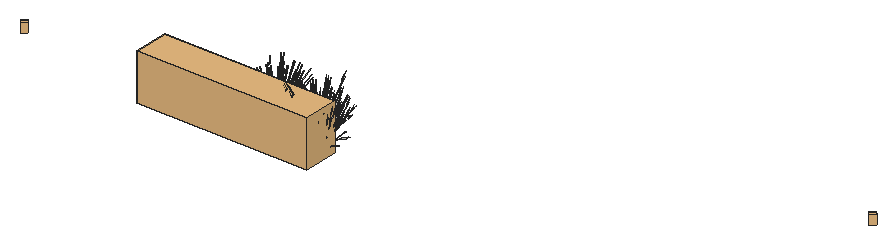
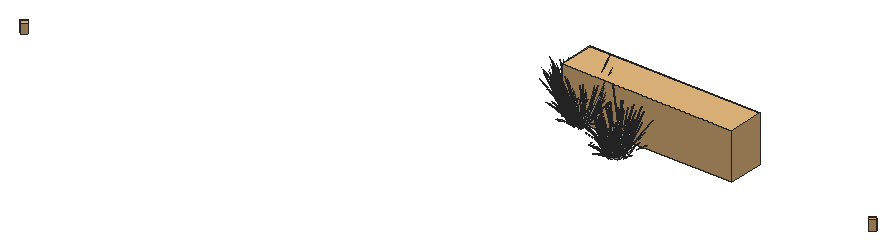
# SketchUp Ruby script. Lengths in inches.
U = 1.inch
M = Sketchup.active_model
def pt(a) = Geom::Point3d.new(a.map { |v| v * U })
def face(e, loops, mat)
  f = e.add_face(loops[0].map { |a| pt(a) })
  loops[1..].each { |l| e.add_face(l.map { |a| pt(a) }).erase! }
  f.material = f.back_material = mat if mat
  f
end
# faces: each face lists its corners as indices into pts; further lists are holes
def faces(e, pts, list, mat = nil) = list.each { |f| face(e, (f[0].is_a?(Array) ? f : [f]).map { |l| l.map { |i| pts[i] } }, mat) }
# xy, xz, yz: faces in a plane at the given z, y or x. An outline is a flat list of corners, or four numbers for a rectangle; further outlines are holes
def ring(l) = l.size == 4 ? [[l[0], l[1]], [l[2], l[1]], [l[2], l[3]], [l[0], l[3]]] : l.each_slice(2).to_a
def flat(e, list, mat, &to3) = list.each { |f| face(e, (f[0].is_a?(Array) ? f : [f]).map { |l| ring(l).map { |u, v| to3.(u, v) } }, mat) }
def xy(e, z, list, mat = nil) = flat(e, list, mat) { |x, y| [x, y, z] }
def xz(e, y, list, mat = nil) = flat(e, list, mat) { |x, z| [x, y, z] }
def yz(e, x, list, mat = nil) = flat(e, list, mat) { |y, z| [x, y, z] }
def lines(e, pts, list) = list.each { |a, b| e.add_line(pt(pts[a]), pt(pts[b])) }
# prism: a flat outline (further loops are holes) pulled along v
def prism(e, loops, v, mat = nil)
  f = face(e, loops, mat); d = Geom::Vector3d.new(v.map { |x| x * U })
  f.pushpull(f.normal.samedirection?(d) ? d.length : -d.length)
end
def box(e, o, s, mat = nil) = prism(e, [[o, [o[0] + s[0], o[1], o[2]], [o[0] + s[0], o[1] + s[1], o[2]], [o[0], o[1] + s[1], o[2]]]], [0, 0, s[2]], mat)
def at(x, y, z, deg = 0) = Geom::Transformation.translation(pt([x, y, z])) * Geom::Transformation.rotation(ORIGIN, Z_AXIS, deg.degrees)
def axes(o, x, y, z) = Geom::Transformation.new([*x, 0, *y, 0, *z, 0, *pt(o).to_a, 1])
def part(name) = M.definitions.add(name)
# library, detail: a bought-in or finely detailed component or shape, given as its bounding box
def library(name, o, s) = part(name).tap { |d| box(d.entities, o, s) }
def detail(e, o, s) = box(e.add_group.entities, o, s)
def put(e, d, t, mat = nil) = e.add_instance(d, t).tap { |i| i.material = mat if mat }
def group(e, t, mat = nil) = e.add_group.tap { |g| g.transformation = t; g.material = mat if mat }.entities
root = M.entities
M.materials.add("LightPink_Translucent").color = [144, 107, 117]
M.materials["LightPink_Translucent"].alpha = 0.75
c1 = part("blade")
p = [[2.15,0.21,22],[0,0.17,0],[0.09,0.45,0],[2.18,0.31,22],[2.29,0.31,22],[0.38,0.45,0],
  [2.48,0.24,33],[2.49,0.24,33],[2.48,0.22,33]]
faces(c1.entities,p,[[0,1,2,3],[4,5,2,3],[6,3,4,7],[8,0,3,6]])
c2 = part("blade with seeds\#1")
put(c2.entities,c1,at(0,0,0))
c3 = part("seeds")
p = [[0.3,-0.1,1.38],[-0.01,-0.03,1.59],[-0.01,-0.03,0.03],[0.14,-0.07,-0.07],[0.29,-0.03,3],[0.15,0.01,3.11]]
faces(c3.entities,p,[[0,1,2,3],[1,0,4,5]],"LightPink_Translucent")
c4 = part("blade with seeds")
put(c4.entities,c1,at(0,0,0))
put(c4.entities,c3,axes([2.4,0.25,30.99],[1.5799,-0.05474,1.17369],[-0.12525,1.92788,0.29478],[-0.07173,-0.02425,1.56792]))
c5 = library("Areca palm plant",[21.56,16.8,2.55],[5.71,6.07,10.56])
c6 = library("Group\#130",[-6.15,-1.2,0],[37.48,180.08,49.04])
c7 = part("PLANTS (1)")
put(c7.entities,c5,axes([-554.71,-75.81,3.93],[0.45017,-0.56191,0],[0.66137,0.52986,0],[0,0,0.72]))
put(c7.entities,c5,axes([38.49,68.02,6.02],[0.45017,-0.56191,0],[0.66137,0.52986,0],[0,0,0.72]))
put(c7.entities,c6,axes([-275.95,-98.77,3.0625],[0,0.79,0],[-0.79,0,0],[0,0,0.79]))
put(root,c2,axes([522.07,92.45,2.78],[-0.61172,0.65782,-0.31925],[-0.57907,-0.75112,0.41216],[-0.08811,0.38163,0.78863]))
put(root,c2,axes([527.67,81.52,2.24],[-0.82131,0.22128,-0.03148],[-0.18882,-1.04586,-0.14272],[0.05207,-0.2184,0.47074]))
put(root,c4,axes([568.41,68.2,4.17],[-1.04497,-0.50058,-0.71045],[0.74264,-0.8772,0.08574],[-0.3786,-0.29889,1.00501]))
put(root,c4,axes([569.55,75.89,4.17],[0.5849,0.8421,-0.71045],[-1.20401,0.4693,0.08574],[0.13677,0.40688,1.00501]))
put(root,c4,axes([566.28,69.43,4.17],[-1.22504,-0.02494,-0.71045],[0.08228,-1.05005,0.08574],[-0.51899,-0.11081,1.00501]))
put(root,c4,axes([575.07,70.45,4.17],[0.64013,-0.81717,-0.71045],[1.12174,0.58074,0.08574],[0.38221,-0.29607,1.00501]))
put(root,c4,axes([575.37,72.51,4.17],[1.07686,-0.45739,-0.71045],[0.60013,0.94154,0.08574],[0.52031,-0.10696,1.00501]))
put(root,c4,axes([573.48,68.78,4.17],[0.03189,-0.95798,-0.71045],[1.34277,0.06434,0.08574],[0.14171,-0.40585,1.00501]))
put(root,c4,axes([574.32,74.41,4.17],[1.22504,0.02494,-0.71045],[-0.08228,1.05005,0.08574],[0.51899,0.11081,1.00501]))
put(root,c4,axes([571.05,67.96,4.17],[-0.5849,-0.8421,-0.71045],[1.20401,-0.4693,0.08574],[-0.13677,-0.40688,1.00501]))
put(root,c2,axes([526.01,85.84,2.19],[-0.16834,0.42944,1.54493],[-0.70619,-0.88871,0.12492],[0.31858,-0.5539,0.66044]))
put(root,c2,axes([521.4,86.39,2.19],[0.33582,0.21526,1.54493],[-0.69497,0.90306,0.12492],[-0.43315,-0.40739,0.66044]))
put(root,c2,axes([524.47,84.9375,2.19],[0.02213,0.47954,1.54493],[-0.95907,-0.31812,0.12492],[0.05932,-0.68338,0.66044]))
put(root,c2,axes([526.99,87.61,2.19],[-0.31369,0.26428,1.54493],[-0.26409,-1.22118,0.12492],[0.49247,-0.276,0.66044]))
put(root,c2,axes([527.15,89.77,2.19],[-0.375,0.0283,1.54493],[0.24877,-1.22643,0.12492],[0.53441,0.07586,0.66044]))
put(root,c2,axes([526.4375,91.74,2.19],[-0.33582,-0.21526,1.54493],[0.69497,-0.90306,0.12492],[0.43315,0.40739,0.66044]))
put(root,c2,axes([525.05,92.99,2.19],[-0.20666,-0.40114,1.54493],[0.95496,-0.33772,0.12492],[0.21583,0.62976,0.66044]))
put(root,c2,axes([525.7,91.52,2.19],[-0.3002,-0.28876,1.54493],[0.81031,-0.72911,0.12492],[0.36902,0.50009,0.66044]))
put(root,c2,axes([520.85,90.51,2.19],[0.31369,-0.26428,1.54493],[0.26409,1.22118,0.12492],[-0.49247,0.276,0.66044]))
put(root,c2,axes([521.83,92.28,2.19],[0.16834,-0.42944,1.54493],[0.70619,0.88871,0.12492],[-0.31858,0.5539,0.66044]))
put(root,c2,axes([523.37,93.19,2.19],[-0.02213,-0.47954,1.54493],[0.95907,0.31812,0.12492],[-0.05932,0.68338,0.66044]))
put(root,c4,axes([569.99,76.06,3.875],[1.20468,0.25962,-0.51099],[-0.41292,0.89013,-0.3958],[0.11046,0.35838,0.97773]))
put(root,c4,axes([573.21,68.46,3.875],[-0.87728,-0.69587,-0.51099],[0.92674,-0.60943,-0.3958],[0.13348,-0.35356,0.97773]))
put(root,c4,axes([567.92,68.22,3.875],[-1.20928,0.24619,-0.51099],[-0.21154,-0.93233,-0.3958],[-0.32481,-0.26718,0.97773]))
put(root,c4,axes([575.59,72.16,3.875],[0.332,-0.94205,-0.51099],[1.13828,0.3229,-0.3958],[0.45829,-0.08638,0.97773]))
put(root,c4,axes([565.875,69.65,3.875],[-0.88986,0.68603,-0.51099],[-0.77932,-0.72471,-0.3958],[-0.45212,-0.10438,0.97773]))
put(root,c4,axes([565.57,73.78,3.875],[0.31482,0.94565,-0.51099],[-1.19224,0.16542,-0.3958],[-0.34166,0.254,0.97773]))
put(root,c4,axes([565.01,71.68,3.875],[-0.332,0.94205,-0.51099],[-1.13828,-0.3229,-0.3958],[-0.45829,0.08638,0.97773]))
put(root,c4,axes([570.61,67.79,3.875],[-1.20468,-0.25962,-0.51099],[0.41292,-0.89013,-0.3958],[-0.11046,-0.35838,0.97773]))
put(root,c4,axes([575.03,70.07,3.875],[-0.31482,-0.94565,-0.51099],[1.19224,-0.16542,-0.3958],[0.34166,-0.254,0.97773]))
put(root,c4,axes([572.68,75.625,3.875],[1.20928,-0.24619,-0.51099],[0.21154,0.93233,-0.3958],[0.32481,0.26718,0.97773]))
put(root,c4,axes([567.12,75.07,4.53],[-0.03189,0.95798,-0.7886],[-1.34277,-0.06434,0.09517],[-0.14171,0.40585,1.11556]))
put(root,c4,axes([567.39,75.38,4.2],[0.87728,0.69587,-0.5672],[-0.92674,0.60943,-0.43934],[-0.13348,0.35356,1.08528]))
put(root,c4,axes([570.91,73.86,2.52],[1.05902,0.41762,1.51261],[-1.03748,0.89969,0.59816],[-0.46471,-0.53324,1.26806]))
put(root,c4,axes([567.42,71.11,2.53],[0.34834,-0.14982,1.77064],[0.12012,1.04605,0.13857],[-0.75452,0.1388,0.63284]))
put(root,c4,axes([566.67,76.41,2.56],[0.02693,-0.53464,1.54345],[1.21102,0.2824,0.21329],[-0.10493,0.5698,0.72882]))
put(root,c4,axes([575.05,74.85,3.72],[0.69728,0.64842,-0.35414],[-0.79619,0.61382,0.4572],[0.40453,0.09339,0.87481]))
put(root,c4,axes([564.31,71.25,3.72],[-1.01846,-0.28891,-0.35414],[0.29705,-0.84289,0.4572],[-0.41005,0.07729,0.87481]))
put(root,c4,axes([564.6875,73.68,3.72],[-1.06674,0.14801,-0.35414],[-0.28168,-0.84611,0.4572],[-0.30569,0.22726,0.87481]))
put(root,c4,axes([576.29,72.59,3.72],[1.01846,0.28891,-0.35414],[-0.29705,0.84289,0.4572],[0.41005,-0.07729,0.87481]))
put(root,c4,axes([568.05,67.53,3.72],[-0.18927,-0.83419,-0.35414],[1.08199,-0.22027,0.4572],[-0.29062,-0.23905,0.87481]))
put(root,c4,axes([566.5625,75.64,3.72],[-0.82919,0.54528,-0.35414],[-0.78493,-0.62262,0.4572],[-0.11943,0.31634,0.87481]))
put(root,c4,axes([575.91,70.16,3.72],[1.06674,-0.14801,-0.35414],[0.28168,0.84611,0.4572],[0.30569,-0.22726,0.87481]))
put(root,c4,axes([569.44,76.6,3.72],[-0.36946,0.79643,-0.35414],[-1.07787,-0.23229,0.4572],[0.09883,0.32066,0.87481]))
put(root,c4,axes([574.04,68.21,3.72],[0.82919,-0.54528,-0.35414],[0.78493,0.62262,0.4572],[0.11943,-0.31634,0.87481]))
put(root,c4,axes([571.16,67.24,3.72],[0.36946,-0.79643,-0.35414],[1.07787,0.23229,0.4572],[-0.09883,-0.32066,0.87481]))
put(root,c4,axes([565.55,69,3.72],[-0.69728,-0.64842,-0.35414],[0.79619,-0.61382,0.4572],[-0.40453,-0.09339,0.87481]))
put(root,c2,axes([527.65,84.23,3.23],[-0.99362,-0.0619,-0.10962],[0.02716,-1.17208,-0.60845],[0.06902,-0.45141,0.92453]))
put(root,c2,axes([523.84,93,3.23],[0.88471,-0.5817,-0.10962],[0.43476,1.03242,-0.60845],[0.11673,0.43507,0.92453]))
put(root,c2,axes([521.91,84.35,3.23],[-0.04841,1.27062,-0.10962],[-0.91657,-0.03473,-0.60845],[-0.353,-0.08826,0.92453]))
put(root,c2,axes([525.8125,82.93,3.23],[-0.88471,0.5817,-0.10962],[-0.43476,-1.03242,-0.60845],[-0.11673,-0.43507,0.92453]))
put(root,c2,axes([528.76,89.23,3.23],[-0.45489,-1.13134,-0.10962],[0.80735,-0.55596,-0.60845],[0.34022,-0.14927,0.92453]))
put(root,c2,axes([522,91.7,3.23],[0.99362,0.0619,-0.10962],[-0.02716,1.17208,-0.60845],[-0.06902,0.45141,0.92453]))
put(root,c2,axes([528.73,86.54,3.23],[-0.8363,-0.68892,-0.10962],[0.4818,-0.99769,-0.60845],[0.23628,-0.3468,0.92453]))
put(root,c2,axes([525.9375,92.96,3.23],[0.53874,-1.06944,-0.10962],[0.78019,0.61612,-0.60845],[0.2712,0.30214,0.92453]))
put(root,c2,axes([520.88,86.7,3.23],[0.45489,1.13134,-0.10962],[-0.80735,0.55596,-0.60845],[-0.34022,0.14927,0.92453]))
put(root,c2,axes([523.71,82.97,3.23],[-0.53874,1.06944,-0.10962],[-0.78019,-0.61612,-0.60845],[-0.2712,-0.30214,0.92453]))
put(root,c2,axes([523.8,85.76,2.73],[-0.50765,0.99901,1.24659],[-0.79039,-1.05487,0.53787],[0.47632,-0.32232,1.20495]))
put(root,c2,axes([524.72,94.22,2.95],[0.12685,0.18879,1.57709],[0.92682,-0.01606,-0.24942],[0.12053,0.43275,0.12648]))
put(root,c2,axes([524.43,79.77,2.95],[-0.14882,-0.16043,1.57709],[-0.91289,0.20534,-0.24942],[-0.17308,-0.40254,0.12648]))
put(root,c2,axes([527.05,83.21,2.95],[-0.01652,-0.24801,1.57709],[-0.75906,-0.68026,-0.24942],[0.1002,-0.44114,0.12648]))
put(root,c2,axes([520.45,83.2,2.95],[-0.19445,0.01116,1.57709],[-0.562,0.94258,-0.24942],[-0.34067,-0.14573,0.12648]))
put(root,c2,axes([528.18,94.1875,2.95],[0.19335,0.02874,1.57709],[0.67262,-0.81555,-0.24942],[0.31807,0.21351,0.12648]))
put(root,c2,axes([530.57,89.49,2.95],[0.15733,-0.14655,1.57709],[0.06181,-1.18266,-0.24942],[0.34698,-0.11893,0.12648]))
put(root,c2,axes([518.77,88.5,2.95],[-0.13699,0.17683,1.57709],[0.08685,1.18009,-0.24942],[-0.32765,0.18834,0.12648]))
put(root,c2,axes([520.28,92.37,2.95],[-0.0069,0.24875,1.57709],[0.68965,0.79195,-0.24942],[-0.14092,0.42256,0.12648]))
put(root,c2,axes([520.86,93.32,2.94],[0.0975,-0.08571,1.59908],[0.87648,0.41319,-0.1511],[0.00634,0.41846,0.28298]))
put(root,c2,axes([518.32,89.71,2.94],[0.11711,0.02157,1.59908],[0.42502,1.06376,-0.1511],[-0.21726,0.31303,0.28298]))
put(root,c2,axes([529.43,87.44,2.94],[-0.11829,-0.00342,1.59908],[-0.52187,-0.99076,-0.1511],[0.18628,-0.34414,0.28298]))
put(root,c2,axes([525.66,96.32,2.94],[0.0262,-0.14755,1.59908],[0.86326,-0.45644,-0.1511],[0.22658,0.30203,0.28298]))
put(root,c2,axes([523.48,80.34,2.94],[-0.00742,0.151,1.59908],[-0.79509,0.62706,-0.1511],[-0.26143,-0.25182,0.28298]))
put(root,c2,axes([528.44,80.61,2.94],[-0.08553,0.10454,1.59908],[-0.91687,-0.22868,-0.1511],[-0.05858,-0.41178,0.28298]))
put(root,c2,axes([530.16,94.28,2.94],[-0.05899,-0.13116,1.59908],[0.39237,-1.08407,-0.1511],[0.32669,0.02548,0.28298]))
put(root,c2,axes([519.75,83.45,2.94],[0.07463,0.11741,1.59908],[-0.25178,1.15035,-0.1511],[-0.32567,0.04164,0.28298]))
put(root,c4,axes([577.13,74.94,3.12],[-0.23455,-0.87059,-0.03492],[1.10861,-0.20015,-0.15832],[0.23151,0.05519,0.52218]))
put(root,c2,axes([527.74,91.58,3.5625],[0.04841,-1.27062,-0.12168],[0.91657,0.03473,-0.67538],[0.353,0.08826,1.02623]))
put(root,c2,axes([520.55,89.41,3.59],[0.93666,0.77159,-0.12278],[-0.53962,1.11741,-0.68147],[-0.26463,0.38842,1.03548]))
put(root,c2,axes([520.58,87.03,2.96],[0.25543,-1.1392,0.43274],[0.83975,0.38955,0.35681],[-0.33023,0.06846,0.89544]))
put(root,c2,axes([527.58,83.74,2.96],[0.64379,0.85247,0.43274],[-0.68369,0.73521,0.35681],[0.11875,-0.39995,0.89544]))
put(root,c2,axes([525.56,82.54,2.96],[0.89085,0.32663,0.43274],[-0.30463,1.07385,0.35681],[-0.05354,-0.4223,0.89544]))
put(root,c2,axes([526.3125,93.13,2.96],[-0.89921,0.28673,0.43274],[-0.15606,-1.12475,0.35681],[0.21148,0.33149,0.89544]))
put(root,c2,axes([528.13,91.49,2.96],[-0.66663,0.82326,0.43274],[-0.57493,-0.87428,0.35681],[0.31276,0.15186,0.89544]))
put(root,c2,axes([521.52,84.44,2.96],[0.66663,-0.82326,0.43274],[0.57493,0.87428,0.35681],[-0.31276,-0.15186,0.89544]))
put(root,c2,axes([524.09,93.39,2.96],[-0.89085,-0.32663,0.43274],[0.30463,-1.07385,0.35681],[0.05354,0.4223,0.89544]))
put(root,c2,axes([523.34,82.8,2.96],[0.89921,-0.28673,0.43274],[0.15606,1.12475,0.35681],[-0.21148,-0.33149,0.89544]))
put(root,c2,axes([528.86,86.0625,2.96],[0.22422,1.14989,0.43274],[-0.87956,0.19957,0.35681],[0.25922,-0.27044,0.89544]))
put(root,c2,axes([520.61,89.65,2.96],[-0.62066,-0.52545,0.05797],[0.36135,-0.74826,0.45634],[-0.19899,0.24191,0.69585]))
put(root,c2,axes([529.13,89.2,2.96],[0.33205,0.8519,0.05797],[-0.60551,0.41697,0.45634],[0.26692,-0.08227,0.69585]))
put(root,c2,axes([523.51,82.58,2.96],[0.4109,-0.79368,0.05797],[0.58514,0.46209,0.45634],[-0.18917,-0.25446,0.69585]))
put(root,c2,axes([525.79,82.46,2.96],[0.66618,-0.42462,0.05797],[0.32607,0.77431,0.45634],[-0.06434,-0.34133,0.69585]))
put(root,c2,axes([521.83,92.11,2.96],[-0.74296,-0.05822,0.05797],[0.02037,-0.87906,0.45634],[-0.07774,0.33673,0.69585]))
put(root,c2,axes([521.58,84.14,2.96],[0.04552,-0.95007,0.05797],[0.68742,0.02605,0.45634],[-0.26332,-0.09941,0.69585]))
put(root,c2,axes([527.82,83.82,2.96],[0.74296,0.05822,0.05797],[-0.02037,0.87906,0.45634],[0.07774,-0.33673,0.69585]))
put(root,c2,axes([526.14,93.35,2.96],[-0.4109,0.79368,0.05797],[-0.58514,-0.46209,0.45634],[0.18917,0.25446,0.69585]))
put(root,c2,axes([520.52,86.73,2.96],[-0.33205,-0.8519,0.05797],[0.60551,-0.41697,0.45634],[-0.26692,0.08227,0.69585]))
put(root,c2,axes([523.86,93.47,2.96],[-0.66618,0.42462,0.05797],[-0.32607,-0.77431,0.45634],[0.06434,0.34133,0.69585]))
put(root,c2,axes([529.04,86.28,2.96],[0.62066,0.52545,0.05797],[-0.36135,0.74826,0.45634],[0.19899,-0.24191,0.69585]))
put(root,c2,axes([528.07,91.79,2.96],[-0.04552,0.95007,0.05797],[-0.68742,-0.02605,0.45634],[0.26332,0.09941,0.69585]))
put(root,c2,axes([528.45,88.89,3.25],[-0.75135,-0.34854,0.31925],[0.21915,-1.01686,-0.41216],[0.30251,-0.09324,0.78863]))
put(root,c2,axes([521.2,87.04,3.25],[0.75135,0.34854,0.31925],[-0.21915,1.01686,-0.41216],[-0.30251,0.09324,0.78863]))
put(root,c2,axes([527.26,84.41,3.25],[-0.61172,0.65782,0.31925],[-0.57907,-0.75112,-0.41216],[0.08811,-0.38163,0.78863]))
put(root,c2,axes([525.55,83.33,3.25],[-0.27256,0.96081,0.31925],[-0.79518,-0.28024,-0.41216],[-0.07291,-0.38684,0.78863]))
put(root,c2,axes([522.39,91.52,3.25],[0.61172,-0.65782,0.31925],[0.57907,0.75112,-0.41216],[-0.08811,0.38163,0.78863]))
put(root,c2,axes([527.6,91.08,3.25],[-0.51441,-0.78225,0.31925],[0.58738,-0.7405,-0.41216],[0.29843,0.11267,0.78863]))
put(root,c2,axes([526.01,92.4375,3.25],[-0.13963,-1.00636,0.31925],[0.79822,-0.26574,-0.41216],[0.2144,0.28839,0.78863]))
put(root,c2,axes([528.32,86.45,3.25],[-0.78697,0.17856,0.31925],[-0.2078,-1.02074,-0.41216],[0.22552,-0.27417,0.78863]))
put(root,c2,axes([523.64,83.49,3.25],[0.13963,1.00636,0.31925],[-0.79822,0.26574,-0.41216],[-0.2144,-0.28839,0.78863]))
put(root,c2,axes([524.1,92.6,3.25],[0.27256,-0.96081,0.31925],[0.79518,0.28024,-0.41216],[0.07291,0.38684,0.78863]))
put(root,c2,axes([522.05,84.85,3.25],[0.51441,0.78225,0.31925],[-0.58738,0.7405,-0.41216],[-0.29843,-0.11267,0.78863]))
put(root,c2,axes([521.33,89.48,3.25],[0.78697,-0.17856,0.31925],[0.2078,1.02074,-0.41216],[-0.22552,0.27417,0.78863]))
put(root,c4,axes([572.55,73.18,3.07],[-0.45521,-0.17844,1.71376],[0.94204,-0.74856,0.13857],[0.58713,0.33769,0.73262]))
put(root,c4,axes([571.97,68.3,3.07],[-0.22818,0.35597,1.71376],[-0.95725,-0.73667,0.13857],[0.43183,-0.45914,0.73262]))
put(root,c4,axes([573.51,71.55,3.07],[-0.50831,0.02346,1.71376],[0.33721,-1.01661,0.13857],[0.72439,0.06288,0.73262]))
put(root,c4,axes([570.67,74.22,3.07],[-0.28013,-0.33252,1.71376],[1.29445,-0.27994,0.13857],[0.29256,0.52202,0.73262]))
put(root,c4,axes([568.39,74.39,3.07],[-0.02999,-0.3975,1.71376],[1.30002,0.26369,0.13857],[-0.08041,0.56647,0.73262]))
put(root,c4,axes([566.3,73.63,3.07],[0.22818,-0.35597,1.71376],[0.95725,0.73667,0.13857],[-0.43183,0.45914,0.73262]))
put(root,c4,axes([564.97,72.17,3.07],[0.42521,-0.21906,1.71376],[0.35798,1.01226,0.13857],[-0.66754,0.22878,0.73262]))
put(root,c4,axes([566.53,72.85,3.07],[0.30609,-0.31822,1.71376],[0.77286,0.85893,0.13857],[-0.53009,0.39116,0.73262]))
put(root,c4,axes([567.6,67.71,3.07],[0.28013,0.33252,1.71376],[-1.29445,0.27994,0.13857],[-0.29256,-0.52202,0.73262]))
put(root,c4,axes([565.72,68.75,3.07],[0.45521,0.17844,1.71376],[-0.94204,0.74856,0.13857],[-0.58713,-0.33769,0.73262]))
put(root,c4,axes([564.76,70.38,3.07],[0.50831,-0.02346,1.71376],[-0.33721,1.01661,0.13857],[-0.72439,-0.06288,0.73262]))
put(root,c7,at(861.08,144.71,0))
put(root,c2,axes([529.07,88.9,3.26],[-0.25543,1.1392,0.48034],[-0.83975,-0.38955,0.39606],[0.33023,-0.06846,0.99394]))
put(root,c2,axes([521.84,92.55,3.29],[-0.72104,-0.95477,0.48466],[0.76573,-0.82343,0.39963],[-0.133,0.44794,1.00289]))
put(root,c2,axes([520.4,89.94,3.29],[-0.25113,-1.28788,0.48466],[0.9851,-0.22351,0.39963],[-0.29033,0.30289,1.00289]))
put(root,c2,axes([531.13,87.52,3.79],[-0.56051,-0.79893,-0.05849],[0.61388,-0.73204,-0.26518],[0.17394,-0.05154,0.87466]))
put(root,c2,axes([528.28,94.72,3.79],[0.2608,-1.0202,-0.05849],[0.8027,0.31383,-0.26518],[0.12187,0.16686,0.87466]))
put(root,c4,axes([574.26,74.92,4.23],[0.06562,-1.05324,-0.1216],[1.2424,0.02879,-0.67495],[0.4785,0.07316,1.02557]))
put(root,c4,axes([564.96,70.875,4.23],[0.6166,0.93779,-0.1216],[-1.09436,0.46085,-0.67495],[-0.46117,0.12373,1.02557]))
put(root,c4,axes([574.13,68.83,4.23],[-1.34686,-0.05131,-0.1216],[0.03681,-0.97156,-0.67495],[0.09356,-0.37418,1.02557]))
put(root,c4,axes([575.64,72.97,4.23],[-0.6166,-0.93779,-0.1216],[1.09436,-0.46085,-0.67495],[0.46117,-0.12373,1.02557]))
put(root,c4,axes([568.96,76.1,4.23],[1.19922,-0.48218,-0.1216],[0.58932,0.85579,-0.67495],[0.15822,0.36063,1.02557]))
put(root,c4,axes([566.34,68.93,4.23],[-0.06562,1.05324,-0.1216],[-1.2424,-0.02879,-0.67495],[-0.4785,-0.07316,1.02557]))
put(root,c4,axes([571.8125,76.06,4.23],[0.73026,-0.88648,-0.1216],[1.05755,0.51071,-0.67495],[0.36761,0.25045,1.02557]))
put(root,c4,axes([565,73.11,4.23],[1.1336,0.57106,-0.1216],[-0.65308,0.827,-0.67495],[-0.32027,0.28747,1.02557]))
put(root,c4,axes([571.64,67.75,4.23],[-1.19922,0.48218,-0.1216],[-0.58932,-0.85579,-0.67495],[-0.15822,-0.36063,1.02557]))
put(root,c4,axes([575.6,70.74,4.23],[-1.1336,-0.57106,-0.1216],[0.65308,-0.827,-0.67495],[0.32027,-0.28747,1.02557]))
put(root,c4,axes([572.64,70.83,3.67],[-1.05895,-0.53811,1.38283],[1.11816,-0.83781,0.59665],[0.34166,0.5049,1.33663]))
put(root,c4,axes([563.67,71.8125,3.91],[-0.20012,0.13446,1.74944],[0.01702,0.98243,-0.27667],[-0.45871,0.12776,0.14031]))
put(root,c4,axes([578.99,71.5,3.91],[0.17006,-0.15775,1.74944],[-0.21766,-0.96766,-0.27667],[0.42669,-0.18347,0.14031]))
put(root,c4,axes([575.34,74.29,3.91],[0.26289,-0.01751,1.74944],[0.72108,-0.8046,-0.27667],[0.46761,0.10621,0.14031]))
put(root,c4,axes([575.35,67.29,3.91],[-0.01183,-0.20612,1.74944],[-0.99913,-0.59572,-0.27667],[0.15447,-0.36112,0.14031]))
put(root,c4,axes([563.7,75.48,3.91],[-0.03046,0.20495,1.74944],[0.86449,0.71297,-0.27667],[-0.22632,0.33716,0.14031]))
put(root,c4,axes([568.68,78.02,3.91],[0.15534,0.16677,1.74944],[1.25362,0.06552,-0.27667],[0.12606,0.3678,0.14031]))
put(root,c4,axes([569.74,65.51,3.91],[-0.18744,-0.14521,1.74944],[-1.25089,0.09206,-0.27667],[-0.19964,-0.34731,0.14031]))
put(root,c4,axes([565.63,67.1,3.91],[-0.26368,-0.00731,1.74944],[-0.83946,0.73103,-0.27667],[-0.44791,-0.14937,0.14031]))
put(root,c4,axes([564.62,67.72,3.9],[0.09085,0.10335,1.77383],[-0.43798,0.92907,-0.16761],[-0.44357,0.00672,0.31391]))
put(root,c4,axes([568.45,65.03,3.9],[-0.02286,0.12414,1.77383],[-1.12758,0.45052,-0.16761],[-0.33182,-0.23029,0.31391]))
put(root,c4,axes([570.86,76.8,3.9],[0.00363,-0.12539,1.77383],[1.0502,-0.55319,-0.16761],[0.36479,0.19745,0.31391]))
put(root,c4,axes([561.45,72.81,3.9],[0.1564,0.02778,1.77383],[0.48382,0.91506,-0.16761],[-0.32016,0.24017,0.31391]))
put(root,c4,axes([578.39,70.49,3.9],[-0.16006,-0.00787,1.77383],[-0.66468,-0.8428,-0.16761],[0.26693,-0.27711,0.31391]))
put(root,c4,axes([578.09,75.76,3.9],[-0.11081,-0.09067,1.77383],[0.2424,-0.97188,-0.16761],[0.43649,-0.06209,0.31391]))
put(root,c4,axes([563.61,77.58,3.9],[0.13903,-0.06253,1.77383],[1.14912,0.41591,-0.16761],[-0.027,0.34629,0.31391]))
put(root,c4,axes([575.09,66.55,3.9],[-0.12446,0.07911,1.77383],[-1.21937,-0.26689,-0.16761],[-0.04414,-0.34521,0.31391]))
put(root,c4,axes([566.47,75.02,4.59],[1.34686,0.05131,-0.13498],[-0.03681,0.97156,-0.74919],[-0.09356,0.37418,1.13838]))
put(root,c4,axes([568.77,67.39,4.62],[-0.81789,0.99285,-0.13619],[-1.18445,-0.572,-0.75594],[-0.41173,-0.28051,1.14864]))
put(root,c4,axes([568.52,67.46,3.92],[0.55698,-0.6579,0.0643],[0.79316,0.38303,0.50621],[-0.25643,-0.21093,0.77189]))
put(root,c4,axes([568.99,76.49,3.92],[-0.90301,0.35198,0.0643],[-0.44199,-0.64184,0.50621],[0.08721,0.28293,0.77189]))
put(root,c4,axes([576.01,70.53,3.92],[0.8413,0.43556,0.0643],[-0.48981,0.62025,0.50621],[0.26973,-0.20053,0.77189]))
put(root,c4,axes([576.14,72.95,3.92],[0.4501,0.70615,0.0643],[-0.82077,0.34564,0.50621],[0.36181,-0.0682,0.77189]))
put(root,c4,axes([565.9,68.75,3.92],[0.06171,-0.78753,0.0643],[0.9318,0.02159,0.50621],[-0.35694,-0.08241,0.77189]))
put(root,c4,axes([574.35,68.48,3.92],[1.00708,0.04826,0.0643],[-0.02761,0.72867,0.50621],[0.10538,-0.27912,0.77189]))
put(root,c4,axes([574.7,75.09,3.92],[-0.06171,0.78753,0.0643],[-0.9318,-0.02159,0.50621],[0.35694,0.08241,0.77189]))
put(root,c4,axes([564.59,73.32,3.92],[-0.8413,-0.43556,0.0643],[0.48981,-0.62025,0.50621],[-0.26973,0.20053,0.77189]))
put(root,c4,axes([571.61,67.36,3.92],[0.90301,-0.35198,0.0643],[0.44199,0.64184,0.50621],[-0.08721,-0.28293,0.77189]))
put(root,c4,axes([564.46,70.9,3.92],[-0.4501,-0.70615,0.0643],[0.82077,-0.34564,0.50621],[-0.36181,0.0682,0.77189]))
put(root,c4,axes([572.08,76.39,3.92],[-0.55698,0.6579,0.0643],[-0.79316,-0.38303,0.50621],[0.25643,0.21093,0.77189]))
put(root,c4,axes([566.25,75.36,3.92],[-1.00708,-0.04826,0.0643],[0.02761,-0.72867,0.50621],[-0.10538,0.27912,0.77189]))
put(root,c4,axes([571.29,67.43,3.93],[1.20755,0.27075,0.48003],[-0.41292,0.89013,0.3958],[-0.07257,-0.35005,0.9933]))
put(root,c4,axes([574.78,74.84,3.93],[-0.90362,0.68241,0.48003],[-0.77932,-0.72471,0.3958],[0.42395,0.12588,0.9933]))
put(root,c4,axes([576.05,72.7,3.93],[-0.34623,0.9443,0.48003],[-1.13828,-0.3229,0.3958],[0.44763,-0.05675,0.9933]))
put(root,c4,axes([564.83,73.5,3.93],[-0.30393,-0.95317,0.48003],[1.19224,-0.16542,0.3958],[-0.35138,0.22417,0.9933]))
put(root,c4,axes([566.57,75.43,3.93],[-0.87265,-0.70663,0.48003],[0.92674,-0.60943,0.3958],[-0.16097,0.33153,0.9933]))
put(root,c4,axes([574.03,68.42,3.93],[0.87265,0.70663,0.48003],[-0.92674,0.60943,0.3958],[0.16097,-0.33153,0.9933]))
put(root,c4,axes([564.55,71.15,3.93],[0.34623,-0.9443,0.48003],[1.13828,0.3229,0.3958],[-0.44763,0.05675,0.9933]))
put(root,c4,axes([575.78,70.35,3.93],[0.30393,0.95317,0.48003],[-1.19224,0.16542,0.3958],[0.35138,-0.22417,0.9933]))
put(root,c4,axes([572.32,76.2,3.93],[-1.21888,0.23767,0.48003],[-0.21154,-0.93233,0.3958],[0.28666,0.27478,0.9933]))
put(root,c4,axes([569.32,75.76,4.24],[0.36946,-0.79643,0.35414],[1.07787,0.23229,-0.4572],[0.09883,0.32066,0.87481]))
put(root,c4,axes([571.28,68.08,4.24],[-0.36946,0.79643,0.35414],[-1.07787,-0.23229,-0.4572],[-0.09883,-0.32066,0.87481]))
put(root,c4,axes([574.07,74.51,4.24],[-0.69728,-0.64842,0.35414],[0.79619,-0.61382,-0.4572],[0.40453,0.09339,0.87481]))
put(root,c4,axes([575.21,72.6875,4.24],[-1.01846,-0.28891,0.35414],[0.29705,-0.84289,-0.4572],[0.41005,-0.07729,0.87481]))
put(root,c4,axes([566.53,69.34,4.24],[0.69728,0.64842,0.35414],[-0.79619,0.61382,-0.4572],[-0.40453,-0.09339,0.87481]))
put(root,c4,axes([567,74.87,4.24],[0.82919,-0.54528,0.35414],[0.78493,0.62262,-0.4572],[-0.11943,0.31634,0.87481]))
put(root,c4,axes([565.56,73.18,4.24],[1.06674,-0.14801,0.35414],[0.28168,0.84611,-0.4572],[-0.30569,0.22726,0.87481]))
put(root,c4,axes([571.91,75.63,4.24],[-0.18927,-0.83419,0.35414],[1.08199,-0.22027,-0.4572],[0.29062,0.23905,0.87481]))
put(root,c4,axes([575.04,70.66,4.24],[-1.06674,0.14801,0.35414],[-0.28168,-0.84611,-0.4572],[0.30569,-0.22726,0.87481]))
put(root,c4,axes([565.39,71.16,4.24],[1.01846,0.28891,0.35414],[-0.29705,0.84289,-0.4572],[-0.41005,0.07729,0.87481]))
put(root,c4,axes([573.6,68.98,4.24],[-0.82919,0.54528,0.35414],[-0.78493,-0.62262,-0.4572],[0.11943,-0.31634,0.87481]))
put(root,c4,axes([568.69,68.21,4.24],[0.18927,0.83419,0.35414],[-1.08199,0.22027,-0.4572],[-0.29062,-0.23905,0.87481]))
put(root,c4,axes([569.31,76.42,4.26],[-1.20755,-0.27075,0.53283],[0.41292,-0.89013,0.43934],[0.07257,0.35005,1.10256]))
put(root,c4,axes([565.44,68.76,4.29],[1.01205,-0.7643,0.53763],[0.87284,0.81167,0.4433],[-0.47482,-0.14098,1.11249]))
put(root,c4,axes([568.2,67.23,4.29],[1.36515,-0.26619,0.53763],[0.23692,1.04421,0.4433],[-0.32106,-0.30775,1.11249]))
put(root,c4,axes([570.77,78.61,4.84],[0.84686,-0.59414,-0.06488],[0.77596,0.65071,-0.29416],[0.05463,0.18438,0.97024]))
put(root,c4,axes([563.14,75.58,4.84],[1.08141,0.27645,-0.06488],[-0.33265,0.85086,-0.29416],[-0.17688,0.12919,0.97024]))
